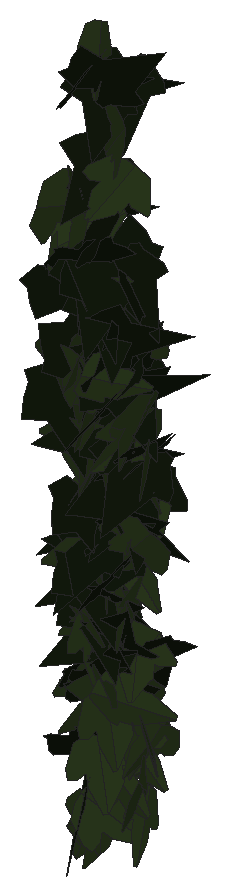
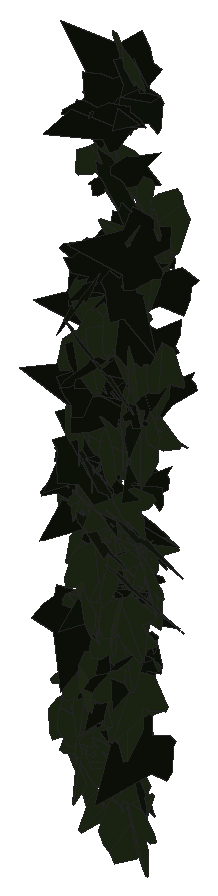
# SketchUp Ruby script. Lengths in inches.
U = 1.inch
M = Sketchup.active_model
def pt(a) = Geom::Point3d.new(a.map { |v| v * U })
def face(e, loops, mat)
  f = e.add_face(loops[0].map { |a| pt(a) })
  loops[1..].each { |l| e.add_face(l.map { |a| pt(a) }).erase! }
  f.material = f.back_material = mat if mat
  f
end
# faces: each face lists its corners as indices into pts; further lists are holes
def faces(e, pts, list, mat = nil) = list.each { |f| face(e, (f[0].is_a?(Array) ? f : [f]).map { |l| l.map { |i| pts[i] } }, mat) }
# xy, xz, yz: faces in a plane at the given z, y or x. An outline is a flat list of corners, or four numbers for a rectangle; further outlines are holes
def ring(l) = l.size == 4 ? [[l[0], l[1]], [l[2], l[1]], [l[2], l[3]], [l[0], l[3]]] : l.each_slice(2).to_a
def flat(e, list, mat, &to3) = list.each { |f| face(e, (f[0].is_a?(Array) ? f : [f]).map { |l| ring(l).map { |u, v| to3.(u, v) } }, mat) }
def xy(e, z, list, mat = nil) = flat(e, list, mat) { |x, y| [x, y, z] }
def xz(e, y, list, mat = nil) = flat(e, list, mat) { |x, z| [x, y, z] }
def yz(e, x, list, mat = nil) = flat(e, list, mat) { |y, z| [x, y, z] }
def lines(e, pts, list) = list.each { |a, b| e.add_line(pt(pts[a]), pt(pts[b])) }
# prism: a flat outline (further loops are holes) pulled along v
def prism(e, loops, v, mat = nil)
  f = face(e, loops, mat); d = Geom::Vector3d.new(v.map { |x| x * U })
  f.pushpull(f.normal.samedirection?(d) ? d.length : -d.length)
end
def box(e, o, s, mat = nil) = prism(e, [[o, [o[0] + s[0], o[1], o[2]], [o[0] + s[0], o[1] + s[1], o[2]], [o[0], o[1] + s[1], o[2]]]], [0, 0, s[2]], mat)
def at(x, y, z, deg = 0) = Geom::Transformation.translation(pt([x, y, z])) * Geom::Transformation.rotation(ORIGIN, Z_AXIS, deg.degrees)
def axes(o, x, y, z) = Geom::Transformation.new([*x, 0, *y, 0, *z, 0, *pt(o).to_a, 1])
def part(name) = M.definitions.add(name)
# library, detail: a bought-in or finely detailed component or shape, given as its bounding box
def library(name, o, s) = part(name).tap { |d| box(d.entities, o, s) }
def detail(e, o, s) = box(e.add_group.entities, o, s)
def put(e, d, t, mat = nil) = e.add_instance(d, t).tap { |i| i.material = mat if mat }
def group(e, t, mat = nil) = e.add_group.tap { |g| g.transformation = t; g.material = mat if mat }.entities
root = M.entities
M.materials.add("efeu1").color = [18, 25, 13]
M.materials.add("efeu2").color = [43, 57, 29]
c1 = part("ivyleaf_9")
p = [[1.54,2.16,1.25],[1.36,2.04,1.19],[-0.21,0.99,0.68],[-0.71,1.11,0.82],[-0.85,0.86,0.67],[-0.8,0.17,0.21],
  [-0.9,-0.01,0.1],[-0.67,-0.16,-0.02],[-0.08,-0.08,-0.05],[-0.03,-0.6,-0.4],[0.65,-0.88,-0.66],[0.83,-0.6,-0.49],
  [1.29,-0.42,-0.43],[1.8125,-0.07,-0.26],[1.21,0.44,0.15]]
faces(c1.entities,p,[[0,1,2,3,4,5,6,7,8,9,10,11,12,13,14]],"efeu1")
c2 = part("ivyleaf_10")
p = [[0,0.5,-0.03],[-0.0625,2.02,-0.43],[-0.19,2.01,-0.46],[-0.54,1.05,-0.29],[-0.52,0.625,-0.18],[-0.83,0.76,-0.28],
  [-1.16,0.64,-0.33],[-1.15,0.33,-0.24],[-0.77,-0.39,0.02],[-0.3,-0.51,0.16],[0.04,-0.48,0.23],[-0.02,2.01,-0.4375],
  [-0.06,2.01,-0.43],[0.04,-0.49,0.23],[0.67,-0.49,0.14],[1.38,0.36,-0.2],[1.375,0.51,-0.24],[0.81,0.65,-0.19],
  [0.62,0.59,-0.15],[0.6,1.09,-0.28],[0.5,1.23,-0.31]]
faces(c2.entities,p,[[0,1,2,3,4,5,6,7,8,9,10],[11,12,0,13,14,15,16,17,18,19,20]],"efeu2")
put(root,c1,axes([508.21,134.79,200.95],[-0.16457,0.48882,0.45651],[-0.18353,0.40594,-0.53149],[-0.68539,-0.22608,0.03271]))
put(root,c1,axes([507.71,135.48,192.72],[-0.72542,-0.17452,-0.17811],[0.1727,0.04363,-0.74611],[0.17988,-0.74569,-0.00197]))
put(root,c2,axes([508.5,135.34,202.44],[0.60178,0.14412,-0.36574],[-0.36536,-0.09634,-0.59851],[-0.18705,0.65182,-0.00759]))
put(root,c2,axes([506.85,135.15,197.21],[-0.78121,0.14761,0.08991],[-0.10578,-0.04943,-0.76456],[-0.15147,-0.72681,0.07026]))
put(root,c2,axes([507.73,135.29,188.5],[-0.66447,0.02331,-0.16284],[-0.16885,0.00927,0.64031],[0.02687,0.6348,-0.00337]))
put(root,c1,axes([507.85,135.62,199.84],[-0.36893,-0.71035,-0.07434],[0.02841,0.06901,-0.80041],[0.71366,-0.36997,-0.00657]))
put(root,c2,axes([507.21,135.13,190.44],[-0.70154,0.2744,-0.0475],[0.05212,0.00292,-0.75298],[-0.27356,-0.70314,-0.02167]))
put(root,c1,axes([508.11,135.8,193.83],[-0.26214,-0.29145,0.56459],[-0.2472,-0.49908,-0.38508],[0.61783,-0.32334,0.08547]))
put(root,c1,axes([507.82,135.17,204.67],[-0.02132,-0.15272,0.71026],[0.75089,-0.08198,0.00183],[0.08596,0.67829,0.16014]))
put(root,c1,axes([506.85,135.01,199.52],[-0.09322,-0.22883,-0.68076],[0.17646,0.63434,-0.25303],[0.72781,-0.18311,-0.02585]))
put(root,c1,axes([506.6,135.4,196.37],[0.06296,-0.73518,-0.27479],[-0.01075,0.27484,-0.73777],[0.78478,0.06275,0.01194]))
put(root,c1,axes([507.52,134.95,200.32],[0.3983,0.56355,-0.11187],[-0.07296,-0.08433,-0.70035],[-0.61531,0.37479,0.01063]))
put(root,c2,axes([508.52,135.07,203.74],[0.37484,-0.37438,-0.46892],[-0.27496,0.37567,-0.52822],[0.57009,0.42735,0.05355]))
put(root,c2,axes([508.36,135.26,191.02],[0.52705,-0.47094,-0.22905],[-0.15288,0.1703,-0.70491],[0.54027,0.5076,0.02398]))
put(root,c1,axes([507.37,135.49,191.76],[0.02645,-0.67132,-0.15846],[0.16622,0.15394,-0.67967],[0.72465,-0.01081,0.16168]))
put(root,c1,axes([507.76,135.45,189.8125],[0.7657,0.11086,-0.00054],[-0.0006,0.00687,0.74627],[0.11973,-0.70895,0.00715]))
put(root,c2,axes([507.93,134.98,197.13],[-0.16966,-0.21148,-0.63969],[0.5058,0.40232,-0.26825],[0.48746,-0.49107,0.05571]))
put(root,c1,axes([507.9,134.89,195.97],[-0.05316,0.64725,0.24969],[-0.0326,0.23844,-0.67498],[-0.74485,-0.05663,0.01172]))
put(root,c2,axes([506.61,134.85,201.26],[-0.10025,-0.20664,-0.71453],[0.31295,0.62296,-0.23558],[0.70884,-0.30426,0.00295]))
put(root,c2,axes([509.01,135.41,192.99],[-0.54963,-0.20402,0.51943],[-0.48789,-0.17826,-0.58627],[0.27092,-0.73493,-0.00199]))
put(root,c1,axes([507.125,135.6,185.66],[-0.36813,0.15585,-0.58706],[0.56026,-0.22268,-0.38972],[-0.29344,-0.62068,-0.00759]))
put(root,c2,axes([506.59,135.69,195.66],[0.20108,-0.21811,-0.64922],[0.41946,-0.48881,0.29809],[-0.578,-0.43061,-0.00953]))
put(root,c1,axes([508.01,135.06,198.07],[0.35988,0.06644,0.64818],[0.66367,0.1044,-0.35326],[-0.13333,0.69899,-0.00885]))
put(root,c1,axes([508.29,135.03,191.88],[-0.07531,0.67122,0.08524],[0.00604,0.08297,-0.70167],[-0.73028,-0.06853,-0.0146]))
put(root,c1,axes([507.42,134.79,193.83],[0.11342,0.40557,0.59603],[0.01844,0.57783,-0.42852],[-0.75803,0.07474,0.07875]))
put(root,c1,axes([507.37,135.63,199.58],[0.19756,-0.77601,-0.0574],[0.00567,0.06066,-0.80051],[0.77811,0.19659,0.02041]))
put(root,c1,axes([507.68,135.86,202.41],[-0.37405,-0.52901,0.25254],[-0.13667,-0.20737,-0.65755],[0.61361,-0.36867,0.00749]))
put(root,c2,axes([507.41,135.02,201.32],[0.04689,-0.08189,-0.78151],[-0.50612,0.58767,-0.09476],[0.64055,0.47033,-0.01767]))
put(root,c2,axes([507.67,135.53,190.49],[-0.24387,-0.69149,0.08203],[-0.00772,-0.08062,-0.75628],[0.75161,-0.22519,0.01885]))
put(root,c1,axes([508.12,135.59,195.52],[-0.6535,0.09027,0.37024],[-0.38884,-0.01027,-0.63372],[-0.07834,-0.70198,0.05688]))
put(root,c1,axes([507.5,135.64,190.86],[-0.06428,-0.65323,-0.18874],[0.15453,0.16598,-0.67011],[0.71572,-0.0945,0.12774]))
put(root,c2,axes([507.26,135.41,195.22],[-0.72899,-0.27439,0.08298],[-0.07047,-0.05127,-0.7574],[0.30046,-0.67775,0.0237]))
put(root,c2,axes([507.7,135.37,190.38],[0.29668,0.68619,-0.03466],[-0.12318,0.01016,-0.76021],[-0.73166,0.27653,0.11393]))
put(root,c2,axes([507.46,135.625,205.67],[0.5924,-0.27428,0.30205],[0.27934,-0.13212,-0.6378],[0.32879,0.60644,-0.00235]))
put(root,c2,axes([507.21,135.51,192.1],[-0.42241,-0.57159,0.04079],[0.04083,-0.07314,-0.71636],[0.61742,-0.38622,0.07528]))
put(root,c1,axes([508.05,135.82,190.25],[-0.65122,-0.21755,0.30891],[-0.28949,-0.13134,-0.66596],[0.27259,-0.65921,0.03074]))
put(root,c2,axes([508.48,135.8,195.41],[0.10948,0.3147,-0.57491],[-0.35979,-0.4506,-0.33032],[-0.58524,0.33589,0.09552]))
put(root,c1,axes([507.97,135.73,199.11],[-0.27907,-0.65499,-0.17986],[0.07182,0.15968,-0.73228],[0.7281,-0.2668,0.00329]))
put(root,c2,axes([507.98,135.39,188.31],[0.3109,0.72514,0.04616],[0.01848,0.0423,-0.78898],[-0.72637,0.31145,-0.00032]))
put(root,c1,axes([507.13,135.49,193.62],[0.15968,-0.62667,-0.36725],[-0.09197,0.34273,-0.66962],[0.7714,0.17058,-0.00381]))
put(root,c1,axes([507.68,135.66,188.45],[0.72889,0.1437,0.19592],[-0.19928,-0.03801,0.71763],[0.16053,-0.69967,0.00125]))
put(root,c1,axes([508.56,136.03,194.78],[-0.32576,-0.66853,0.20551],[-0.08486,-0.18725,-0.74366],[0.69424,-0.33659,0.00553]))
put(root,c2,axes([508.68,135.8125,196.21],[0.12311,-0.7276,0.27853],[0.04703,-0.27453,-0.73794],[0.77767,0.13179,0.00054]))
put(root,c2,axes([506.84,135.68,191.67],[0.62145,-0.43734,0.09137],[0.07656,-0.05192,-0.75166],[0.47564,0.57977,0.0016]))
put(root,c1,axes([508.03,135.74,196.76],[0.35551,0.42955,0.54046],[-0.38076,-0.38509,0.55653],[0.57587,-0.51979,0.03432]))
put(root,c2,axes([508.36,135.8,199.03],[-0.39178,-0.34339,0.46323],[-0.29259,-0.35779,-0.51634],[0.53229,-0.44942,0.05713]))
put(root,c2,axes([506.72,135.51,199.99],[0.12146,0.6881,-0.04305],[-0.01072,-0.04032,-0.72511],[-0.74441,0.11285,0.00342]))
put(root,c2,axes([506.9,135.36,200.24],[0.42004,0.04198,-0.60556],[0.60483,0.17071,0.40183],[0.17801,-0.67909,0.06358]))
put(root,c1,axes([507.29,135.02,204.53],[0.1674,0.43266,0.53561],[0.06926,0.51659,-0.47142],[-0.72313,0.14963,0.07884]))
put(root,c1,axes([507.14,135.34,197.11],[-0.39201,-0.27899,0.61375],[0.50555,0.35937,0.47612],[-0.49135,0.59234,0.00022]))
put(root,c1,axes([508.43,135.72,192.47],[-0.54334,0.10343,0.57262],[-0.55926,0.12351,-0.55297],[-0.16067,-0.77965,-0.01164]))
put(root,c2,axes([507.17,135.61,197.26],[0.22544,-0.74177,-0.16767],[-0.02495,0.16757,-0.77489],[0.76007,0.22551,0.02429]))
put(root,c2,axes([507.27,135.51,191.7],[-0.64439,0.40383,0.02809],[-0.02272,0.01664,-0.76047],[-0.40417,-0.64478,-0.00203]))
put(root,c2,axes([508.78,135.96,189.76],[-0.09171,-0.11572,0.63377],[-0.41113,-0.4759,-0.14915],[0.52892,-0.38999,-0.00605]))
put(root,c2,axes([508.48,135.89,195.71],[-0.17282,-0.71901,0.22616],[0.00032,-0.2321,-0.73765],[0.75374,-0.16476,0.05217]))
put(root,c2,axes([507.95,135.64,198.1],[-0.53574,-0.46533,-0.04269],[0.03285,0.02758,-0.70735],[0.50344,-0.49698,0.00072]))
put(root,c2,axes([508.04,135.34,188.56],[-0.29025,-0.21236,-0.73377],[0.64245,0.35679,-0.35738],[0.41325,-0.70382,0.04023]))
put(root,c1,axes([507.56,136.03,204.38],[-0.25134,-0.62089,0.01062],[-0.00395,-0.00953,-0.68959],[0.67064,-0.23275,-0.00008]))
put(root,c2,axes([508.1875,135.76,193.07],[0.5273,-0.40482,-0.03862],[-0.03008,0.0246,-0.65961],[0.43802,0.48903,0.0012]))
put(root,c2,axes([507.57,135.77,198.3],[0.03735,-0.79445,-0.01493],[0.00064,0.01498,-0.79533],[0.79459,0.03733,0.00134]))
put(root,c2,axes([507.46,136.05,195.08],[0.08372,-0.74234,0.35722],[0.03837,-0.35515,-0.74704],[0.82292,0.09209,-0.00151]))
put(root,c2,axes([508.54,135.74,189.94],[0.62583,0.31814,-0.02097],[-0.02621,0.00232,-0.68736],[-0.34328,0.57982,0.01425]))
put(root,c1,axes([507.53,135.41,190.97],[0.77977,0.13254,0.09326],[0.08174,0.08229,-0.76027],[-0.15227,0.72288,0.06944]))
put(root,c2,axes([507.84,135.61,194.56],[-0.21122,0.61606,0.06111],[-0.01574,0.05702,-0.6722],[-0.66818,-0.19609,-0.00348]))
put(root,c1,axes([507.4,135.3125,189.27],[0.19552,0.6289,0.15812],[0.04545,0.1461,-0.68061],[-0.69729,0.18586,-0.00003]))
put(root,c2,axes([508.69,135.97,193.7],[0.35612,0.18958,-0.50995],[-0.45991,-0.24308,-0.39557],[-0.33292,0.53859,0.00097]))
put(root,c1,axes([508.14,135.77,199.89],[-0.25473,-0.28565,-0.57015],[0.40328,0.40179,-0.38481],[0.53207,-0.44129,0.0187]))
put(root,c2,axes([507.43,135.75,186.75],[0.48492,0.56207,0.0754],[0.06219,0.04677,-0.74799],[-0.60889,0.45241,-0.01635]))
put(root,c2,axes([507.38,135.6,195.93],[0.19062,-0.66633,-0.3782],[-0.02625,0.38382,-0.68946],[0.76573,0.17903,0.07051]))
put(root,c2,axes([508.45,136.08,191.29],[0.21743,-0.66895,0.25142],[0.06901,-0.24192,-0.70334],[0.71129,0.22796,-0.00861]))
put(root,c2,axes([508.18,135.72,192.03],[0.49913,0.14996,0.47179],[0.44384,0.19714,-0.5032],[-0.26319,0.61686,0.04613]))
put(root,c1,axes([507.4375,135.93,192.92],[-0.67756,0.32495,-0.0151],[-0.04686,-0.11486,-0.72377],[-0.34816,-0.61694,0.1268]))
put(root,c1,axes([508.24,135.51,193.15],[0.65759,0.21833,0.15405],[0.14901,0.05408,-0.67269],[-0.24287,0.6243,0.0044]))
put(root,c1,axes([508.32,136.08,194.01],[-0.73804,-0.12735,-0.1659],[0.15997,0.04825,-0.74868],[0.13473,-0.75492,-0.01986]))
put(root,c1,axes([507.96,135.96,196.08],[0.4337,0.40912,0.43432],[-0.37614,-0.23951,0.59232],[0.50712,-0.52753,0.0679]))
put(root,c2,axes([507.99,136.1,190.71],[0.0288,-0.7296,0.21948],[0.00958,-0.21927,-0.73017],[0.76184,0.03034,0.00089]))
put(root,c1,axes([507.85,135.9,197.06],[0.10964,-0.72856,-0.40087],[0.03367,0.4079,-0.73213],[0.83089,0.07961,0.08257]))
put(root,c1,axes([507.39,135.49,188.58],[0.55365,0.42225,0.05255],[0.03627,0.0387,-0.69066],[-0.45785,0.51367,0.00883]))
put(root,c1,axes([507.75,136.09,202.66],[-0.5602,0.26995,-0.32076],[0.25799,-0.20514,-0.60455],[-0.35971,-0.56754,0.06594]))
put(root,c1,axes([508.22,135.9,194.09],[-0.59306,0.48941,-0.02115],[0.01693,-0.01271,-0.76892],[-0.48957,-0.5933,-0.00097]))
put(root,c2,axes([507.2,135.89,187.82],[-0.1629,-0.69789,-0.14303],[0.00538,0.14551,-0.71613],[0.71237,-0.16068,-0.0273]))
put(root,c1,axes([508.25,135.8,199.49],[0.54081,-0.30848,-0.33093],[-0.27663,0.19037,-0.61114],[0.39061,0.56193,0.02537]))
put(root,c1,axes([508.12,136.14,199.51],[-0.21896,0.07996,0.65867],[-0.68934,-0.01432,-0.21062],[-0.01148,-0.66484,0.08376]))
put(root,c2,axes([507.07,136.5,184.23],[-0.12948,-0.28298,-0.65862],[-0.19843,-0.62898,0.30926],[-0.68883,0.23438,0.03472]))
put(root,c2,axes([507.79,135.91,192.97],[-0.75433,0.15028,-0.02924],[0.02237,-0.03726,-0.76848],[-0.15146,-0.75398,0.03215]))
put(root,c1,axes([507.3,136.1,191.375],[-0.68472,0.26929,0.03447],[-0.07874,-0.08796,-0.70729],[-0.28224,-0.62874,0.11371]))
put(root,c2,axes([507.56,136.19,186.08],[-0.34611,-0.03458,-0.6433],[0.56799,-0.36099,-0.28618],[-0.30401,-0.63507,0.1977]))
put(root,c2,axes([508.41,136.18,185.53],[0.65198,-0.31371,0.18344],[0.15933,-0.09186,-0.7234],[0.32661,0.67103,-0.01328]))
put(root,c1,axes([508.41,136.34,194.02],[-0.24027,-0.71737,-0.11227],[0.01246,0.11417,-0.75615],[0.72599,-0.23938,-0.02418]))
put(root,c2,axes([507.86,135.76,190.93],[-0.2557,0.66394,0.23671],[-0.14306,0.19768,-0.70901],[-0.6902,-0.28695,0.05927]))
put(root,c1,axes([508.2,136.2,192.66],[-0.65996,0.31647,-0.2085],[0.13879,-0.18779,-0.72433],[-0.35265,-0.66615,0.10514]))
put(root,c1,axes([507.375,136.375,188.72],[-0.12413,-0.67779,-0.00565],[-0.0038,0.00611,-0.71495],[0.73203,-0.1149,-0.00467]))
put(root,c1,axes([506.71,135.67,186.86],[0.63757,0.39277,0.06094],[0.03826,0.05247,-0.73701],[-0.42718,0.59092,0.02494]))
put(root,c2,axes([507.3,136.11,189.76],[-0.68729,-0.15889,0.23378],[-0.20512,-0.14256,-0.69991],[0.19449,-0.71183,0.08799]))
put(root,c2,axes([507.92,136.25,192.97],[-0.67948,0.1576,-0.31858],[0.21778,-0.35857,-0.64189],[-0.28089,-0.65925,0.27296]))
put(root,c2,axes([508.58,135.96,187.74],[-0.42243,0.51125,0.02101],[-0.01403,0.0155,-0.66946],[-0.5524,-0.39135,0.00094]))
put(root,c2,axes([508.52,136.51,187.28],[0.01285,-0.37102,0.5408],[0.0666,-0.51699,-0.3851],[0.68667,0.05708,0.02723]))
put(root,c2,axes([507.88,135.97,193.04],[-0.64233,0.4254,0.00059],[0.00049,0.00181,-0.77043],[-0.4254,-0.64233,-0.00178]))
put(root,c2,axes([506.86,136.07,184.71],[0.61372,-0.325,-0.21094],[-0.13723,0.1824,-0.67421],[0.39032,0.57514,0.09462]))
put(root,c2,axes([507.81,136.16,190.17],[0.45027,-0.00643,-0.5438],[-0.56405,0.02829,-0.43345],[0.02822,0.66815,0.01312]))
put(root,c2,axes([507.28,136.28,195.03],[-0.10429,0.03801,-0.66683],[0.61131,-0.30144,-0.10724],[-0.32789,-0.57409,0.01216]))
put(root,c2,axes([507.36,135.6875,185.3],[0.18985,0.51236,0.58931],[0.21428,0.54901,-0.54636],[-0.75092,0.2862,-0.00692]))
put(root,c2,axes([508.62,136.3125,187.32],[-0.36939,-0.4889,0.27654],[-0.15714,-0.22269,-0.62048],[0.58015,-0.37161,0.00801]))
put(root,c1,axes([508.65,135.79,189.75],[0.36606,0.59495,-0.03779],[-0.02918,-0.02642,-0.71203],[-0.64308,0.33986,0.0108]))
put(root,c2,axes([508.67,135.92,195.09],[0.41926,-0.58988,-0.4084],[-0.06919,0.43757,-0.70304],[0.71411,0.38871,0.17166]))
put(root,c2,axes([508.23,136.23,197.63],[-0.48145,-0.4493,0.14771],[-0.10335,-0.10512,-0.65822],[0.49831,-0.45591,0.0062]))
put(root,c1,axes([508.23,135.53,194.65],[0.39553,0.5153,0.42065],[0.15215,0.40633,-0.64083],[-0.64756,0.41022,0.10636]))
put(root,c1,axes([508.46,135.97,197.38],[-0.49085,0.51373,0.33176],[-0.24697,0.22266,-0.71017],[-0.55946,-0.54902,0.02242]))
put(root,c2,axes([507.15,136.36,193.48],[0.45764,0.52911,-0.30696],[-0.19627,-0.23608,-0.69955],[-0.57936,0.49792,-0.00548]))
put(root,c2,axes([507.89,136.21,187.05],[-0.57339,-0.0925,-0.46736],[0.49547,-0.11492,-0.53909],[-0.00569,-0.68601,0.15332]))
put(root,c2,axes([508.33,136.17,193.99],[-0.61017,0.45764,-0.12235],[0.06468,-0.11716,-0.76079],[-0.46928,-0.61119,0.05423]))
put(root,c2,axes([507.09,136.55,190.01],[-0.2256,0.17842,0.64508],[0.5003,-0.41251,0.28565],[0.48536,0.50814,0.00539]))
put(root,c2,axes([507.07,136.26,190.49],[-0.55869,-0.1477,0.3045],[-0.28816,-0.12837,-0.55761],[0.20592,-0.58038,0.04585]))
put(root,c2,axes([508.52,135.85,186.16],[0.09357,-0.53219,-0.58167],[-0.07499,0.57709,-0.54006],[0.78482,0.11859,0.01775]))
put(root,c2,axes([508.27,136.12,188.18],[-0.21303,-0.6232,-0.20394],[0.07985,0.18223,-0.67964],[0.70106,-0.21013,0.01544]))
put(root,c2,axes([506.93,136.11,188.41],[-0.52522,-0.46966,-0.21119],[0.17433,0.12169,-0.70416],[0.48456,-0.55285,0.02442]))
put(root,c2,axes([507.96,136.54,188.55],[0.22907,-0.51541,0.34771],[0.1226,-0.31473,-0.57949],[0.65207,0.24023,-0.01319]))
put(root,c1,axes([506.4375,135.95,200.59],[0.35507,0.04279,0.59748],[0.61095,0.10113,-0.34452],[-0.11768,0.65415,0.01418]))
put(root,c1,axes([507.06,136.29,199.76],[-0.34631,0.52187,-0.29406],[0.16881,-0.23579,-0.63694],[-0.6184,-0.35661,-0.0092]))
put(root,c1,axes([507.86,135.9,196.23],[0.28074,0.51226,-0.44128],[0.21328,0.37558,0.5974],[0.68599,-0.32641,-0.00514]))
put(root,c1,axes([507.57,135.8,204.2],[0.42279,0.25725,0.49286],[0.38428,0.31678,-0.48452],[-0.43757,0.52676,0.05069]))
put(root,c1,axes([508.19,136.31,193.22],[-0.63077,0.3657,0.23302],[-0.25301,0.02367,-0.72203],[-0.35217,-0.67202,0.10137]))
put(root,c1,axes([507.61,136.51,204.53],[-0.39456,-0.46473,-0.311],[0.26823,0.18216,-0.60997],[0.53317,-0.43556,0.07672]))
put(root,c1,axes([508.39,136.14,194.5],[-0.27727,0.71307,-0.10855],[-0.05041,-0.13517,-0.75916],[-0.71952,-0.26531,0.09502]))
put(root,c2,axes([507.78,136.41,191.85],[-0.42026,-0.62854,0.07317],[0.03358,-0.10987,-0.75089],[0.63189,-0.41219,0.08857]))
